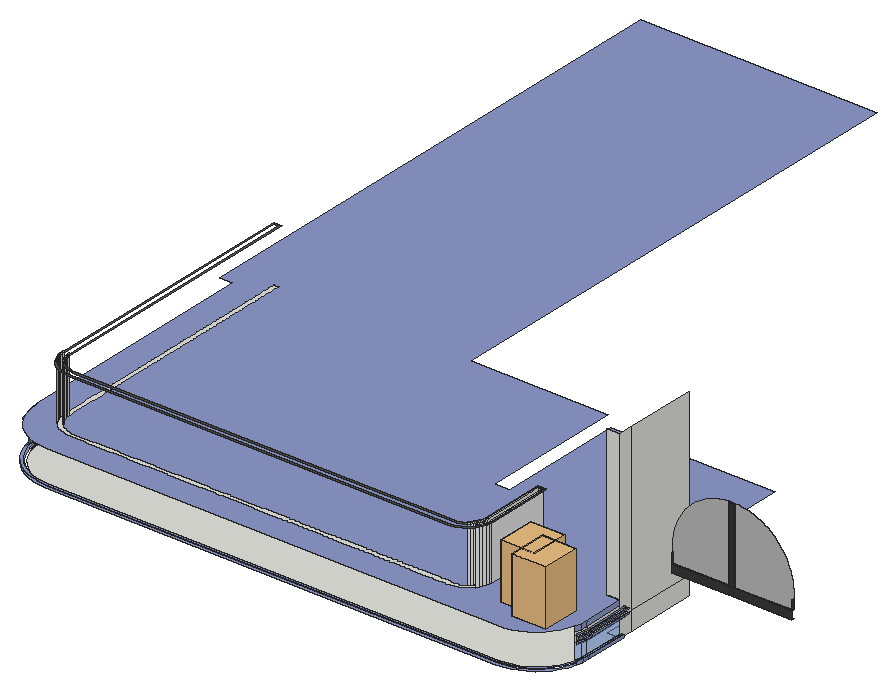
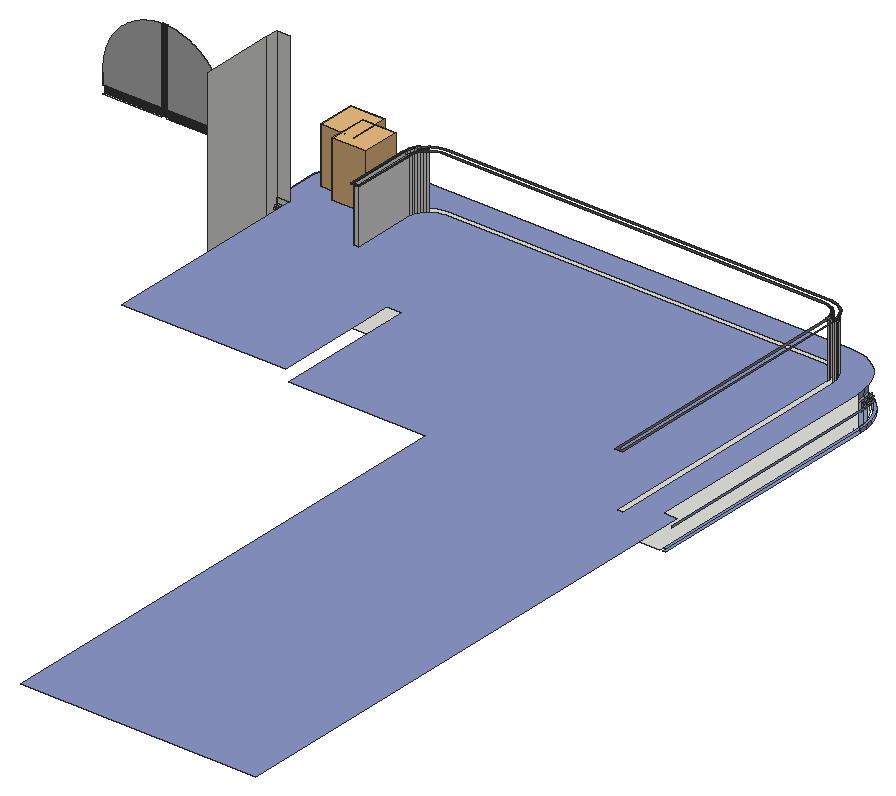
# SketchUp Ruby script. Lengths in inches.
U = 1.inch
M = Sketchup.active_model
def pt(a) = Geom::Point3d.new(a.map { |v| v * U })
def face(e, loops, mat)
  f = e.add_face(loops[0].map { |a| pt(a) })
  loops[1..].each { |l| e.add_face(l.map { |a| pt(a) }).erase! }
  f.material = f.back_material = mat if mat
  f
end
# faces: each face lists its corners as indices into pts; further lists are holes
def faces(e, pts, list, mat = nil) = list.each { |f| face(e, (f[0].is_a?(Array) ? f : [f]).map { |l| l.map { |i| pts[i] } }, mat) }
# xy, xz, yz: faces in a plane at the given z, y or x. An outline is a flat list of corners, or four numbers for a rectangle; further outlines are holes
def ring(l) = l.size == 4 ? [[l[0], l[1]], [l[2], l[1]], [l[2], l[3]], [l[0], l[3]]] : l.each_slice(2).to_a
def flat(e, list, mat, &to3) = list.each { |f| face(e, (f[0].is_a?(Array) ? f : [f]).map { |l| ring(l).map { |u, v| to3.(u, v) } }, mat) }
def xy(e, z, list, mat = nil) = flat(e, list, mat) { |x, y| [x, y, z] }
def xz(e, y, list, mat = nil) = flat(e, list, mat) { |x, z| [x, y, z] }
def yz(e, x, list, mat = nil) = flat(e, list, mat) { |y, z| [x, y, z] }
def lines(e, pts, list) = list.each { |a, b| e.add_line(pt(pts[a]), pt(pts[b])) }
# prism: a flat outline (further loops are holes) pulled along v
def prism(e, loops, v, mat = nil)
  f = face(e, loops, mat); d = Geom::Vector3d.new(v.map { |x| x * U })
  f.pushpull(f.normal.samedirection?(d) ? d.length : -d.length)
end
def box(e, o, s, mat = nil) = prism(e, [[o, [o[0] + s[0], o[1], o[2]], [o[0] + s[0], o[1] + s[1], o[2]], [o[0], o[1] + s[1], o[2]]]], [0, 0, s[2]], mat)
def at(x, y, z, deg = 0) = Geom::Transformation.translation(pt([x, y, z])) * Geom::Transformation.rotation(ORIGIN, Z_AXIS, deg.degrees)
def axes(o, x, y, z) = Geom::Transformation.new([*x, 0, *y, 0, *z, 0, *pt(o).to_a, 1])
def part(name) = M.definitions.add(name)
# library, detail: a bought-in or finely detailed component or shape, given as its bounding box
def library(name, o, s) = part(name).tap { |d| box(d.entities, o, s) }
def detail(e, o, s) = box(e.add_group.entities, o, s)
def put(e, d, t, mat = nil) = e.add_instance(d, t).tap { |i| i.material = mat if mat }
def group(e, t, mat = nil) = e.add_group.tap { |g| g.transformation = t; g.material = mat if mat }.entities
root = M.entities
M.materials.add("0326 AP 7207 CLASSIC PURPLE").color = [140, 152, 201]
M.materials.add("[Color M06]").color = [86, 86, 86]
M.materials.add("[Color M07]").color = [58, 58, 58]
M.materials.add("[Mirror 01]").color = [185, 185, 185]
M.materials.add("[Mirror 02]").color = [229, 229, 229]
M.materials.add("[Translucent Glass Blue]").color = [100, 149, 237]
M.materials["[Translucent Glass Blue]"].alpha = 0.5
c1 = library("Ficus elastica Belize 002",[-7.92,-8.8125,0.01],[22.14,24.73,36.43])
xy(root,252,[[45.79,28.41,41.61,28.68,37.51,29.49,33.55,30.84,29.8,32.6875,26.32,35.01,23.18,37.77,20.42,40.91,18.1,44.39,16.25,48.14,14.9,52.1,14.09,56.21,13.8125,60.38,13.8125,220.92,37.41,220.92,37.41,86.25,65.51,86.25,65.51,95.25,169.65,95.25,169.65,86.25,190.41,86.25,190.41,133.75,228.58,133.75,228.58,138.25,330.09,138.25,330.09,133.75,364.41,133.75,364.41,86.25,371.25,86.25,371.25,59.13,370.98,55.0625,370.2,51.13,368.91,47.33,367.14,43.74,364.91,40.4,362.79,37.98,362.27,37.39,359.25,34.74,355.92,32.52,352.32,30.74,348.53,29.45,344.6,28.67,340.52,28.41],[37.41,86.25,46.41,142.75],[46.41,86.25,65.51,95.25],[169.65,86.25,181.41,95.25],[181.41,86.25,190.41,95.25],
  [364.41,86.25,370.72,86.25,370.72,86.78,372.66,86.78,372.66,87.53,373.41,87.53,373.41,142.75,364.41,142.75],[370.72,86.25,372.66,86.78],[372.66,86.25,373.41,86.78],[372.66,86.78,373.41,87.53],[46.41,95.25,181.41,142.75],
  [181.41,95.25,190.41,142.75],[190.41,133.75,228.58,142.75],[330.09,133.75,364.41,142.75]])
xy(root,252,[[45.79,24.97,41.16,25.28,36.62,26.18,32.24,27.67,28.08,29.72,24.23,32.29,20.75,35.34,17.7,38.83,15.125,42.68,13.08,46.83,11.59,51.22,10.68,55.76,10.38,60.38,10.38,220.92,12.4,220.92,12.4,60.38,12.6875,56.02,13.54,51.74,14.94,47.6,16.875,43.6875,19.3,40.06,22.18,36.77,25.46,33.89,29.09,31.47,33.01,29.54,37.15,28.13,41.43,27.28,45.79,26.99,340.57,26.99,344.78,27.27,348.89,28.09,352.87,29.4375,356.63,31.29,360.11,33.62,363.27,36.39,363.85,37.05,366.03,39.54,368.36,43.03,370.22,46.79,371.57,50.76,372.39,54.88,372.66,59.09,372.66,86.25,373.41,86.25,373.41,87.53,374.68,87.53,374.68,59.02,374.39,54.61,373.52,50.24,372.09,46.02,370.12,42.02,367.64,38.31,365.37,35.72,364.7,34.96,361.35,32.02,357.64,29.54,353.64,27.57,349.42,26.13,345.04,25.26,340.64,24.97]],"0326 AP 7207 CLASSIC PURPLE")
xy(root,254.0625,[[45.79,24.97,340.64,24.97,345.04,25.26,349.42,26.13,353.64,27.57,357.64,29.54,361.35,32.02,364.7,34.96,365.37,35.72,367.64,38.31,370.12,42.02,372.09,46.02,373.52,50.24,374.39,54.61,374.68,59.02,374.68,87.53,373.41,87.53,373.41,59.0625,373.125,54.78,372.29,50.57,370.91,46.51,369.01,42.66,366.625,39.09,364.41,36.56,363.8,35.86,360.57,33.03,357,30.65,353.15,28.75,349.09,27.37,344.88,26.53,340.59,26.25,45.79,26.25,41.33,26.54,36.95,27.41,32.73,28.85,28.72,30.82,25.01,33.3,21.65,36.25,18.71,39.6,16.23,43.31,14.25,47.32,12.82,51.55,11.95,55.92,11.66,60.38,11.66,220.92,10.38,220.92,10.38,60.38,10.68,55.76,11.59,51.22,13.08,46.83,15.125,42.68,17.7,38.83,20.75,35.34,24.23,32.29,28.08,29.72,32.24,27.67,36.62,26.18,41.16,25.28]],"0326 AP 7207 CLASSIC PURPLE")
xy(root,274.4375,[[45.79,43.83,43.625,43.97,41.5,44.4,39.45,45.09,37.51,46.05,35.71,47.25,34.09,48.68,32.66,50.31,31.46,52.11,30.5,54.05,29.8,56.1,29.38,58.22,29.24,60.38,29.24,232.52,32.41,232.52,32.41,60.38,32.52,58.63,32.86,56.92,33.42,55.26,34.2,53.6875,35.17,52.23,36.32,50.92,37.64,49.76,39.1,48.79,40.67,48.02,42.32,47.45,44.04,47.11,45.79,47,294.72,47,296.39,47.11,298.03,47.43,299.61,47.97,301.11,48.71,302.5,49.64,303.75,50.74,304.85,52,305.78,53.38,306.52,54.88,307.06,56.47,307.38,58.1,307.49,59.77,307.49,101.2,310.66,101.2,310.66,59.625,310.53,57.6875,310.125,55.64,309.46,53.67,308.53,51.8,307.49,50.24,307.375,50.0625,306,48.49,304.43,47.12,302.69,45.96,300.82,45.04,298.85,44.37,296.8,43.96,294.87,43.83]])
xy(root,274.4375,[[[45.79,26.25,340.59,26.25,344.88,26.53,349.09,27.37,353.15,28.75,357,30.65,360.57,33.03,363.8,35.86,364.41,36.56,366.625,39.09,369.01,42.66,370.91,46.51,372.29,50.57,373.125,54.78,373.41,59.0625,373.41,86.25,364.41,86.25,364.41,224.35,257.02,224.35,257.02,141.25,247.2,141.25,247.2,233.75,157.41,233.75,157.41,566.25,2.97,566.25,2.97,220.92,11.66,220.92,11.66,60.38,11.95,55.92,12.82,51.55,14.25,47.32,16.23,43.31,18.71,39.6,21.65,36.25,25.01,33.3,28.72,30.82,32.73,28.85,36.95,27.41,41.33,26.54],[45.79,43.83,43.625,43.97,41.5,44.4,39.45,45.09,37.51,46.05,35.71,47.25,34.09,48.68,32.66,50.31,31.46,52.11,30.5,54.05,29.8,56.1,29.38,58.22,29.24,60.38,29.24,232.52,32.41,232.52,32.41,60.38,32.52,58.63,32.86,56.92,33.42,55.26,34.2,53.6875,35.17,52.23,36.32,50.92,37.64,49.76,39.1,48.79,40.67,48.02,42.32,47.45,44.04,47.11,45.79,47,294.72,47,296.39,47.11,298.03,47.43,299.61,47.97,301.11,48.71,302.5,49.64,303.75,50.74,304.85,52,305.78,53.38,306.52,54.88,307.06,56.47,307.38,58.1,307.49,59.77,307.49,101.2,310.66,101.2,310.66,59.625,310.53,57.6875,310.125,55.64,309.46,53.67,308.53,51.8,307.49,50.24,307.375,50.0625,306,48.49,304.43,47.12,302.69,45.96,300.82,45.04,298.85,44.37,296.8,43.96,294.87,43.83]]],"0326 AP 7207 CLASSIC PURPLE")
xy(root,299.08,[[403.41,90.75,440.73,91.75],[444.31,90.75,482.61,91.75]])
xy(root,304.37,[[403.41,90.75,440.73,91.75],[444.31,90.75,482.61,91.75]],"[Color M07]")
xy(root,310.4375,[[[45.79,42.77,43.49,42.92,41.23,43.37,39.05,44.11,36.98,45.13,35.07,46.41,33.33,47.93,31.81,49.66,30.53,51.57,29.52,53.64,28.78,55.82,28.33,58.08,28.18,60.38,28.18,233.58,33.47,233.58,33.47,60.38,33.57,58.77,33.89,57.19,34.41,55.67,35.12,54.22,36.01,52.88,37.08,51.67,38.29,50.61,39.63,49.71,41.07,49,42.6,48.48,44.18,48.17,45.79,48.0625,294.72,48.0625,296.25,48.16,297.75,48.46,299.2,48.95,300.58,49.63,301.85,50.48,303,51.49,304.01,52.64,304.86,53.92,305.54,55.29,306.03,56.74,306.33,58.24,306.43,59.77,306.43,102.26,311.72,102.26,311.72,59.59,311.59,57.55,311.15,55.37,310.44,53.26,309.46,51.26,308.375,49.65,308.22,49.41,306.75,47.74,305.08,46.27,304.84,46.11,303.23,45.04,301.23,44.05,299.125,43.34,296.94,42.9,294.9,42.77],[45.79,43.83,294.87,43.83,296.8,43.96,298.85,44.37,300.82,45.04,302.69,45.96,304.43,47.12,306,48.49,307.375,50.0625,307.49,50.24,308.53,51.8,309.46,53.67,310.125,55.64,310.53,57.6875,310.66,59.625,310.66,101.2,307.49,101.2,307.49,59.77,307.38,58.1,307.06,56.47,306.52,54.88,305.78,53.38,304.85,52,303.75,50.74,302.5,49.64,301.11,48.71,299.61,47.97,298.03,47.43,296.39,47.11,294.72,47,45.79,47,44.04,47.11,42.32,47.45,40.67,48.02,39.1,48.79,37.64,49.76,36.32,50.92,35.17,52.23,34.2,53.6875,33.42,55.26,32.86,56.92,32.52,58.63,32.41,60.38,32.41,232.52,29.24,232.52,29.24,60.38,29.38,58.22,29.8,56.1,30.5,54.05,31.46,52.11,32.66,50.31,34.09,48.68,35.71,47.25,37.51,46.05,39.45,45.09,41.5,44.4,43.625,43.97]]],"[Color M06]")
xz(root,86.25,[[371.25,252,372.66,252.5625],[364.41,264,373.41,264.4375],[364.41,264.4375,373.41,268.875],[364.41,268.875,373.41,270.75],[364.41,270.75,373.41,274.4375],
  [364.41,274.4375,373.41,372]])
xz(root,86.78,[[373.41,252,373.9375,254.0625]])
xz(root,87.53,[[373.41,252,374.68,254.0625]])
xz(root,88.07,[[366.22,264.4375,375.22,265.875],[366.22,265.875,375.22,266.8125],[366.22,266.8125,375.22,268.875],[366.22,268.875,375.22,269.625],[366.22,269.625,375.22,270.75]])
xz(root,89.22,[[367.375,265.875,376.375,266.8125],[367.375,268.875,376.375,269.625]])
xz(root,90.75,[[403.41,299.08,440.73,304.37],[440.73,299.08,444.31,304.37],[444.31,299.08,482.61,304.37],[440.73,304.37,444.31,304.37,444.31,353.68,440.73,353.61]],"[Color M07]")
xz(root,91.75,[[403.41,304.37,440.73,304.37,440.73,353.61,444.31,353.68,443.01,353.7,441.71,353.68,440.41,353.61,439.12,353.51,437.82,353.36,436.54,353.17,435.26,352.93,433.99,352.66,432.73,352.34,431.48,351.99,430.24,351.59,429.01,351.15,427.81,350.67,426.61,350.15,425.4375,349.6,424.28,349,423.14,348.37,422.03,347.7,420.9375,347,419.87,346.26,418.82,345.48,417.81,344.67,416.82,343.83,415.85,342.96,414.92,342.05,414.02,341.12,413.14,340.15,412.3,339.16,411.5,338.14,410.72,337.1,409.98,336.03,409.28,334.93,408.61,333.82,407.98,332.68,407.39,331.52,406.83,330.35,406.32,329.16,405.84,327.95,405.4,326.72,405.01,325.48,404.65,324.23,404.34,322.97,404.0625,321.7,403.83,320.42,403.64,319.13,403.5,317.84,403.41,316.76],[444.31,304.37,482.61,304.37,482.61,316.76,482.52,317.84,482.38,319.13,482.1875,320.42,481.96,321.7,481.68,322.97,481.37,324.23,481.01,325.48,480.62,326.72,480.18,327.95,479.7,329.16,479.1875,330.35,478.63,331.52,478.04,332.68,477.41,333.82,476.74,334.93,476.04,336.03,475.3,337.1,474.53,338.14,473.72,339.16,472.875,340.15,472,341.12,471.1,342.05,470.17,342.96,469.2,343.83,468.21,344.67,467.2,345.48,466.15,346.26,465.08,347,463.99,347.7,462.875,348.37,461.74,349,460.58,349.6,459.41,350.15,458.21,350.67,457.01,351.15,455.78,351.59,454.54,351.99,453.29,352.34,452.03,352.66,450.76,352.93,449.48,353.17,448.2,353.36,446.9,353.51,445.61,353.61,444.31,353.68]],"[Mirror 01]")
xz(root,101.2,[[307.49,274.4375,310.66,310.4375],[307.49,310.4375,310.66,311.125]])
xz(root,102.26,[[306.43,310.4375,311.72,311.125]])
yz(root,8.6875,[[60.38,265.875,217.95,266.8125]],"0326 AP 7207 CLASSIC PURPLE")
yz(root,306.43,[[59.77,310.4375,102.26,311.125]],"[Color M06]")
yz(root,307.49,[[59.77,310.4375,101.2,311.125]])
yz(root,307.49,[[59.77,274.4375,101.2,310.4375]],"[Mirror 02]")
yz(root,310.66,[[59.625,310.4375,101.2,311.125]])
yz(root,310.66,[[59.625,274.4375,101.2,310.4375]],"[Mirror 02]")
yz(root,311.72,[[59.59,310.4375,102.26,311.125]],"[Color M06]")
yz(root,371.25,[[59.13,252,84.09,252.375],[84.09,252,86.25,252.5625],[59.13,252.375,84.09,252.5625]])
yz(root,372.66,[[59.09,252,86.25,252.5625]])
yz(root,373.41,[[86.25,252,86.78,254.0625],[87.53,252,95.25,252,95.25,264,86.25,264,86.25,254.0625,87.53,254.0625],[86.78,252,87.53,254.0625],[95.25,252,142.75,264],[86.25,264,95.25,372],
  [95.25,264,142.75,372],[59.0625,264.4375,86.25,268.875],[59.0625,268.875,86.25,270.75]])
yz(root,373.41,[[59.0625,270.75,86.25,274.4375]],"0326 AP 7207 CLASSIC PURPLE")
yz(root,373.41,[[59.0625,254.0625,86.25,264.4375]],"[Translucent Glass Blue]")
yz(root,374.68,[[59.02,252,87.53,254.0625]],"0326 AP 7207 CLASSIC PURPLE")
yz(root,375.22,[[59,265.875,88.07,266.8125],[59,268.875,88.07,269.625]])
yz(root,375.22,[[59,264.4375,88.07,265.875],[59,266.8125,88.07,268.875],[59,269.625,88.07,270.75]],"0326 AP 7207 CLASSIC PURPLE")
yz(root,376.375,[[58.97,265.875,89.22,266.8125],[58.97,268.875,89.22,269.625]],"0326 AP 7207 CLASSIC PURPLE")
yz(root,403.41,[[90.75,304.37,91.75,311]],"[Color M07]")
yz(root,440.73,[[90.75,304.37,91.75,353.61]],"[Color M07]")
yz(root,444.31,[[90.75,304.37,91.75,353.68]],"[Color M07]")
yz(root,482.61,[[90.75,304.37,91.75,311]],"[Color M07]")
p = [[373.52,50.24,252],[374.39,54.61,252],[374.39,54.61,254.0625],[373.52,50.24,254.0625],[372.39,54.88,252],[371.57,50.76,252],
  [371.57,50.76,252.5625],[372.39,54.88,252.5625],[370.2,51.13,252],[370.98,55.0625,252],[370.98,55.0625,252.375],[370.2,51.13,252.375],
  [10.68,55.76,252],[11.59,51.22,252],[11.59,51.22,254.0625],[10.68,55.76,254.0625],[13.54,51.74,252],[12.6875,56.02,252],
  [12.6875,56.02,252.5625],[13.54,51.74,252.5625],[14.09,56.21,252],[14.9,52.1,252],[14.9,52.1,252.375],[14.09,56.21,252.375],
  [374.68,59.02,252],[374.68,59.02,254.0625],[372.66,59.09,252],[372.66,59.09,252.5625],[371.25,59.13,252],[371.25,59.13,252.375],
  [10.38,60.38,252],[10.38,60.38,254.0625],[12.4,60.38,252],[12.4,60.38,252.5625],[13.8125,60.38,252],[13.8125,60.38,252.375],
  [370.2,51.13,252.5625],[370.98,55.0625,252.5625],[14.09,56.21,252.5625],[14.9,52.1,252.5625],[371.25,59.13,252.5625],[13.8125,60.38,252.5625],
  [373.125,54.78,254.0625],[373.125,54.78,264.4375],[372.29,50.57,264.4375],[372.29,50.57,254.0625],[12.82,51.55,254.0625],[12.82,51.55,264.4375],
  [11.95,55.92,264.4375],[11.95,55.92,254.0625],[373.41,59.0625,254.0625],[373.41,59.0625,264.4375],[11.66,60.38,264.4375],[11.66,60.38,254.0625],
  [374.93,54.54,265.875],[374.05,50.1,265.875],[374.05,50.1,264.4375],[374.93,54.54,264.4375],[373.125,54.78,268.875],[372.29,50.57,268.875],
  [11.07,51.08,265.875],[10.15,55.6875,265.875],[10.15,55.6875,264.4375],[11.07,51.08,264.4375],[12.82,51.55,268.875],[11.95,55.92,268.875],
  [375.22,59,265.875],[375.22,59,264.4375],[373.41,59.0625,268.875],[9.84,60.38,265.875],[9.84,60.38,264.4375],[11.66,60.38,268.875],
  [375.16,49.8,265.875],[376.08,54.39,265.875],[376.08,54.39,266.8125],[375.16,49.8,266.8125],[374.93,54.54,266.8125],[374.05,50.1,266.8125],
  [9,55.54,265.875],[9.95,50.78,265.875],[9.95,50.78,266.8125],[9,55.54,266.8125],[11.07,51.08,266.8125],[10.15,55.6875,266.8125],
  [376.375,58.97,265.875],[376.375,58.97,266.8125],[375.22,59,266.8125],[8.6875,60.38,265.875],[8.6875,60.38,266.8125],[9.84,60.38,266.8125],
  [374.05,50.1,268.875],[374.93,54.54,268.875],[10.15,55.6875,268.875],[11.07,51.08,268.875],[375.22,59,268.875],[9.84,60.38,268.875],
  [375.16,49.8,268.875],[376.07,54.39,268.875],[376.07,54.39,269.625],[375.16,49.8,269.625],[374.93,54.54,269.625],[374.05,50.1,269.625],
  [373.125,54.78,270.75],[372.29,50.57,270.75],[9.01,55.54,268.875],[9.95,50.78,268.875],[9.95,50.78,269.625],[9.01,55.54,269.625],
  [11.07,51.08,269.625],[10.15,55.6875,269.625],[12.82,51.55,270.75],[11.95,55.92,270.75],[376.375,58.97,268.875],[376.375,58.97,269.625],
  [375.22,59,269.625],[373.41,59.0625,270.75],[8.69,60.38,268.875],[8.69,60.38,269.625],[9.84,60.38,269.625],[11.66,60.38,270.75],
  [374.05,50.1,270.75],[374.93,54.54,270.75],[10.15,55.6875,270.75],[11.07,51.08,270.75],[375.22,59,270.75],[9.84,60.38,270.75],
  [373.125,54.78,274.4375],[372.29,50.57,274.4375],[12.82,51.55,274.4375],[11.95,55.92,274.4375],[373.41,59.0625,274.4375],[11.66,60.38,274.4375],
  [303.75,50.74,274.4375],[302.5,49.64,274.4375],[302.5,49.64,310.4375],[303.75,50.74,310.4375],[37.64,49.76,274.4375],[36.32,50.92,274.4375],
  [36.32,50.92,310.4375],[37.64,49.76,310.4375],[307.49,50.24,274.4375],[308.53,51.8,274.4375],[308.53,51.8,310.4375],[307.49,50.24,310.4375],
  [31.46,52.11,274.4375],[32.66,50.31,274.4375],[32.66,50.31,310.4375],[31.46,52.11,310.4375],[304.85,52,274.4375],[304.85,52,310.4375],
  [35.17,52.23,274.4375],[35.17,52.23,310.4375],[309.46,53.67,274.4375],[309.46,53.67,310.4375],[305.78,53.38,274.4375],[305.78,53.38,310.4375],
  [30.5,54.05,274.4375],[30.5,54.05,310.4375],[34.2,53.6875,274.4375],[34.2,53.6875,310.4375],[306.52,54.88,274.4375],[306.52,54.88,310.4375],
  [33.42,55.26,274.4375],[33.42,55.26,310.4375],[310.125,55.64,274.4375],[310.125,55.64,310.4375],[29.8,56.1,274.4375],[29.8,56.1,310.4375],
  [307.06,56.47,274.4375],[307.06,56.47,310.4375],[32.86,56.92,274.4375],[32.86,56.92,310.4375],[310.53,57.6875,274.4375],[310.53,57.6875,310.4375],
  [29.38,58.22,274.4375],[29.38,58.22,310.4375],[307.38,58.1,274.4375],[307.38,58.1,310.4375],[32.52,58.63,274.4375],[32.52,58.63,310.4375],
  [310.66,59.625,274.4375],[310.66,59.625,310.4375],[307.49,59.77,274.4375],[307.49,59.77,310.4375],[29.24,60.38,274.4375],[29.24,60.38,310.4375],
  [32.41,60.38,274.4375],[32.41,60.38,310.4375],[303.75,50.74,311.125],[302.5,49.64,311.125],[30.53,51.57,310.4375],[31.81,49.66,310.4375],
  [31.81,49.66,311.125],[30.53,51.57,311.125],[39.63,49.71,310.4375],[38.29,50.61,310.4375],[38.29,50.61,311.125],[39.63,49.71,311.125],
  [308.375,49.65,310.4375],[309.46,51.26,310.4375],[309.46,51.26,311.125],[308.375,49.65,311.125],[37.64,49.76,311.125],[36.32,50.92,311.125],
  [307.375,50.0625,310.4375],[307.375,50.0625,311.125],[307.49,50.24,311.125],[308.53,51.8,311.125],[31.46,52.11,311.125],[32.66,50.31,311.125],
  [303,51.49,310.4375],[301.85,50.48,310.4375],[301.85,50.48,311.125],[303,51.49,311.125],[37.08,51.67,310.4375],[37.08,51.67,311.125],
  [304.85,52,311.125],[35.17,52.23,311.125],[310.44,53.26,310.4375],[310.44,53.26,311.125],[304.01,52.64,310.4375],[304.01,52.64,311.125],
  [29.52,53.64,310.4375],[29.52,53.64,311.125],[36.01,52.88,310.4375],[36.01,52.88,311.125],[309.46,53.67,311.125],[305.78,53.38,311.125],
  [30.5,54.05,311.125],[34.2,53.6875,311.125],[304.86,53.92,310.4375],[304.86,53.92,311.125],[35.12,54.22,310.4375],[35.12,54.22,311.125],
  [311.15,55.37,310.4375],[311.15,55.37,311.125],[306.52,54.88,311.125],[28.78,55.82,310.4375],[28.78,55.82,311.125],[33.42,55.26,311.125],
  [310.125,55.64,311.125],[305.54,55.29,310.4375],[305.54,55.29,311.125],[29.8,56.1,311.125],[34.41,55.67,310.4375],[34.41,55.67,311.125],
  [307.06,56.47,311.125],[32.86,56.92,311.125],[306.03,56.74,310.4375],[306.03,56.74,311.125],[311.59,57.55,310.4375],[311.59,57.55,311.125],
  [310.53,57.6875,311.125],[33.89,57.19,310.4375],[33.89,57.19,311.125],[28.33,58.08,310.4375],[28.33,58.08,311.125],[29.38,58.22,311.125],
  [307.38,58.1,311.125],[306.33,58.24,310.4375],[306.33,58.24,311.125],[32.52,58.63,311.125],[33.57,58.77,310.4375],[33.57,58.77,311.125],
  [311.72,59.59,310.4375],[311.72,59.59,311.125],[310.66,59.625,311.125],[28.18,60.38,310.4375],[28.18,60.38,311.125],[307.49,59.77,311.125],
  [29.24,60.38,311.125],[306.43,59.77,310.4375],[306.43,59.77,311.125],[32.41,60.38,311.125],[33.47,60.38,310.4375],[33.47,60.38,311.125],
  [15.26,60.38,252],[15.26,60.38,252.375],[369.8,59.18,252],[369.8,59.18,252.375],[369.8,84.09,252],[369.8,84.09,252.375],
  [373.41,59.0625,252],[11.66,60.38,252],[310.67,59.77,274.4375],[373.9375,59.05,254.0625],[373.9375,86.78,254.0625],[373.65,54.71,254.0625],
  [372.8,50.43,254.0625],[373.9375,59.05,252],[11.125,60.38,252],[11.125,60.38,254.0625]]
faces(root,p,[[0,1,2,3],[12,13,14,15],[1,24,25,2],[30,12,15,31],[54,55,56,57],[60,61,62,63],[66,54,57,67],[61,69,70,62],
  [72,73,74,75],[78,79,80,81],[73,84,85,74],[87,78,81,88],[90,77,76,91],[92,83,82,93],[91,76,86,94],[95,89,83,92],
  [96,97,98,99],[104,105,106,107],[97,112,113,98],[116,104,107,117],[120,101,100,121],[122,109,108,123],[121,100,114,124],[125,118,109,122],
  [126,127,103,102],[128,129,111,110],[130,126,102,115],[129,131,119,111]],"0326 AP 7207 CLASSIC PURPLE")
faces(root,p,[[4,5,6,7],[8,9,10,11],[16,17,18,19],[20,21,22,23],[26,4,7,27],[9,28,29,10],[17,32,33,18],[34,20,23,35],
  [36,11,10,37],[38,23,22,39],[37,10,29,40],[41,35,23,38],[43,58,59,44],[47,64,65,48],[51,68,58,43],[48,65,71,52],
  [55,54,76,77],[61,60,82,83],[54,66,86,76],[69,61,83,89],[90,91,100,101],[59,58,102,103],[92,93,108,109],[65,64,110,111],
  [91,94,114,100],[58,68,115,102],[95,92,109,118],[71,65,111,119],[134,135,188,189],[194,195,196,197],[138,139,202,203],[143,204,205,206],
  [142,143,206,207],[146,147,208,209],[195,214,215,196],[135,149,216,188],[151,138,203,217],[214,224,225,215],[153,142,207,226],[149,155,227,216],
  [147,157,228,208],[159,151,217,229],[224,232,233,225],[155,161,236,227],[163,159,229,239],[165,153,226,240],[157,167,243,228],[232,244,245,233],
  [161,169,246,236],[171,163,239,247],[173,165,240,252],[244,253,254,245],[167,175,257,243],[169,177,258,246],[179,171,247,261],[253,262,263,254],
  [181,173,252,266],[177,183,269,258],[175,185,270,257],[187,179,261,273],[262,274,275,263]])
faces(root,p,[[42,43,44,45],[46,47,48,49],[50,51,43,42],[49,48,52,53]],"[Translucent Glass Blue]")
faces(root,p,[[132,133,134,135],[136,137,138,139],[140,141,142,143],[144,145,146,147],[148,132,135,149],[137,150,151,138],[141,152,153,142],[154,148,149,155],
  [156,144,147,157],[150,158,159,151],[160,154,155,161],[158,162,163,159],[152,164,165,153],[166,156,157,167],[168,160,161,169],[162,170,171,163],
  [164,172,173,165],[174,166,167,175],[176,168,169,177],[170,178,179,171],[172,180,181,173],[182,176,177,183],[184,174,175,185],[178,186,187,179]],"[Mirror 02]")
faces(root,p,[[190,191,192,193],[198,199,200,201],[210,211,212,213],[199,218,219,200],[220,210,213,221],[222,190,193,223],[230,220,221,231],[218,234,235,219],
  [237,222,223,238],[241,230,231,242],[248,241,242,249],[234,250,251,235],[255,237,238,256],[259,248,249,260],[250,264,265,251],[267,255,256,268],
  [271,259,260,272]],"[Color M06]")
lines(root,p,[[276,277],[278,279],[280,281],[282,50],[283,53],[180,284],[285,286],[287,285],[288,287],[289,285],[290,291]])
put(root,c1,at(348.31,47.68,274.4375))
put(root,c1,at(334.6,55.25,274.4375))
